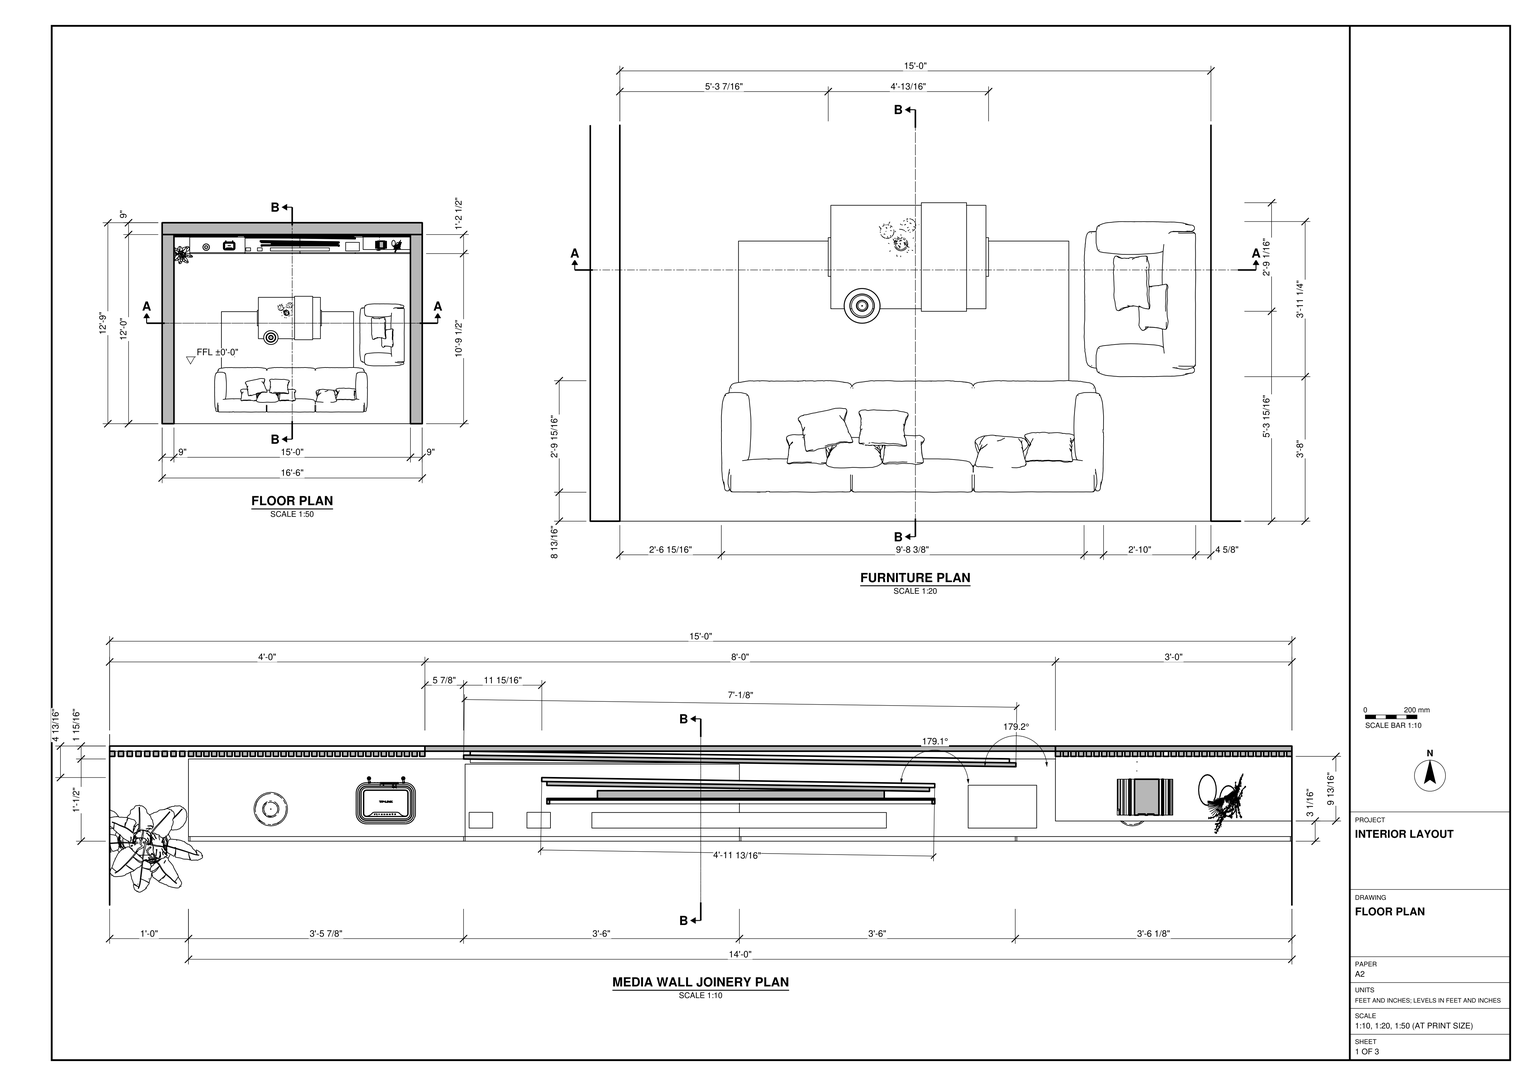
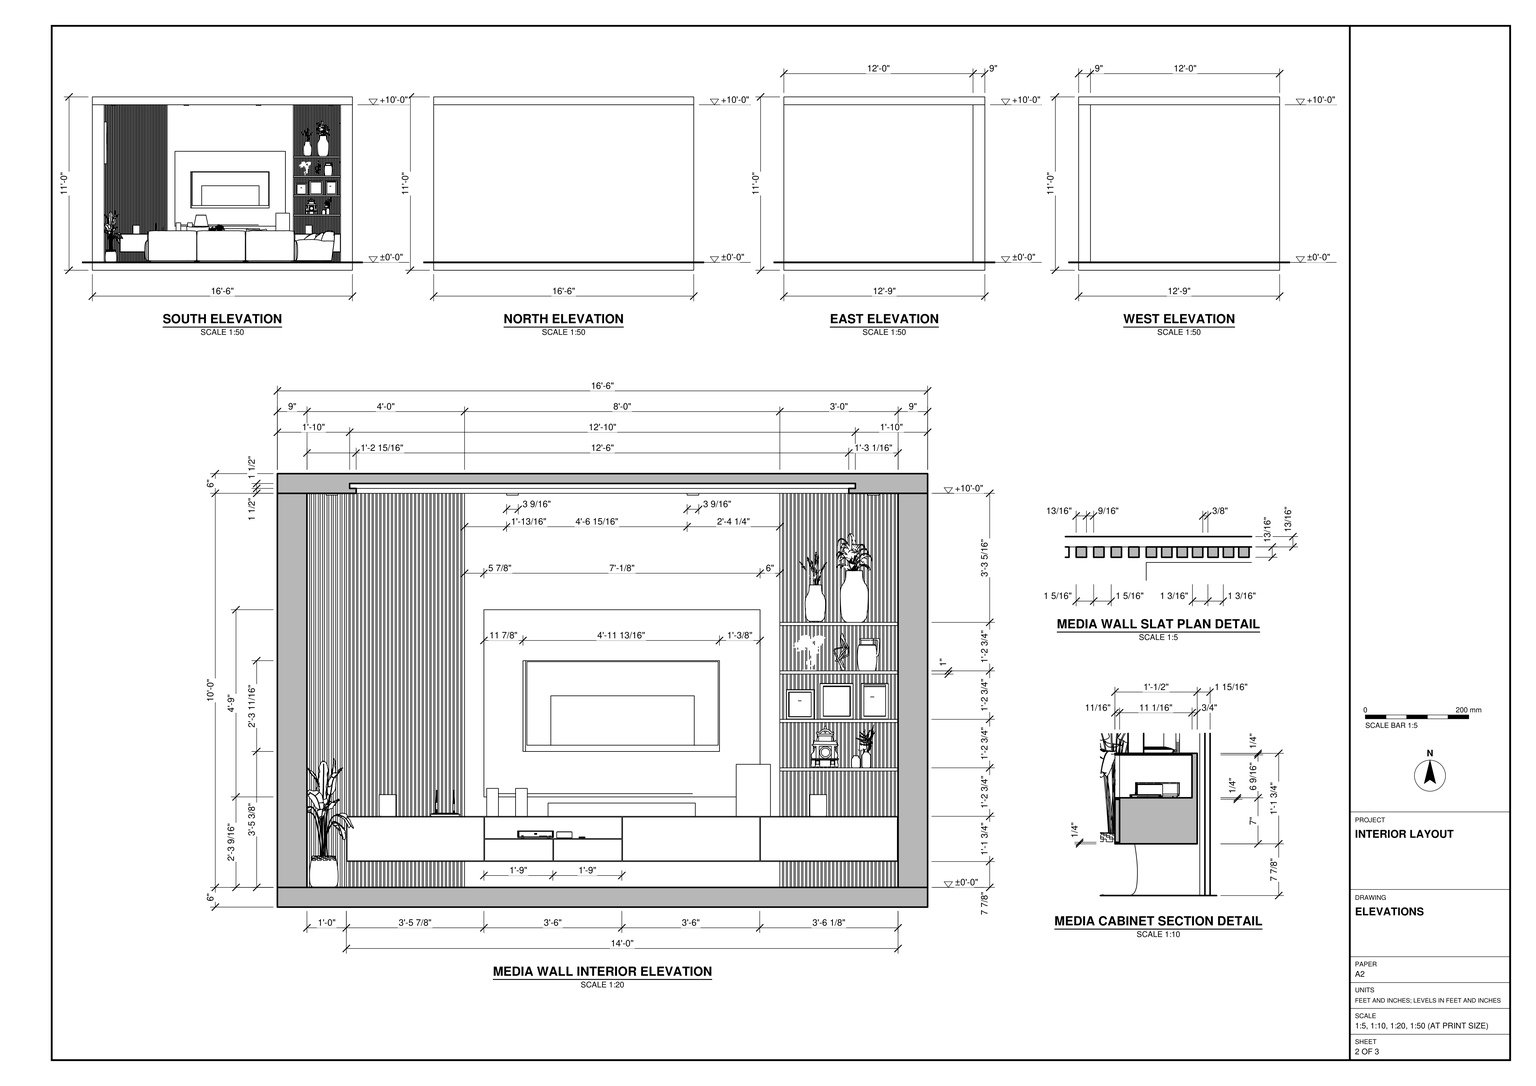
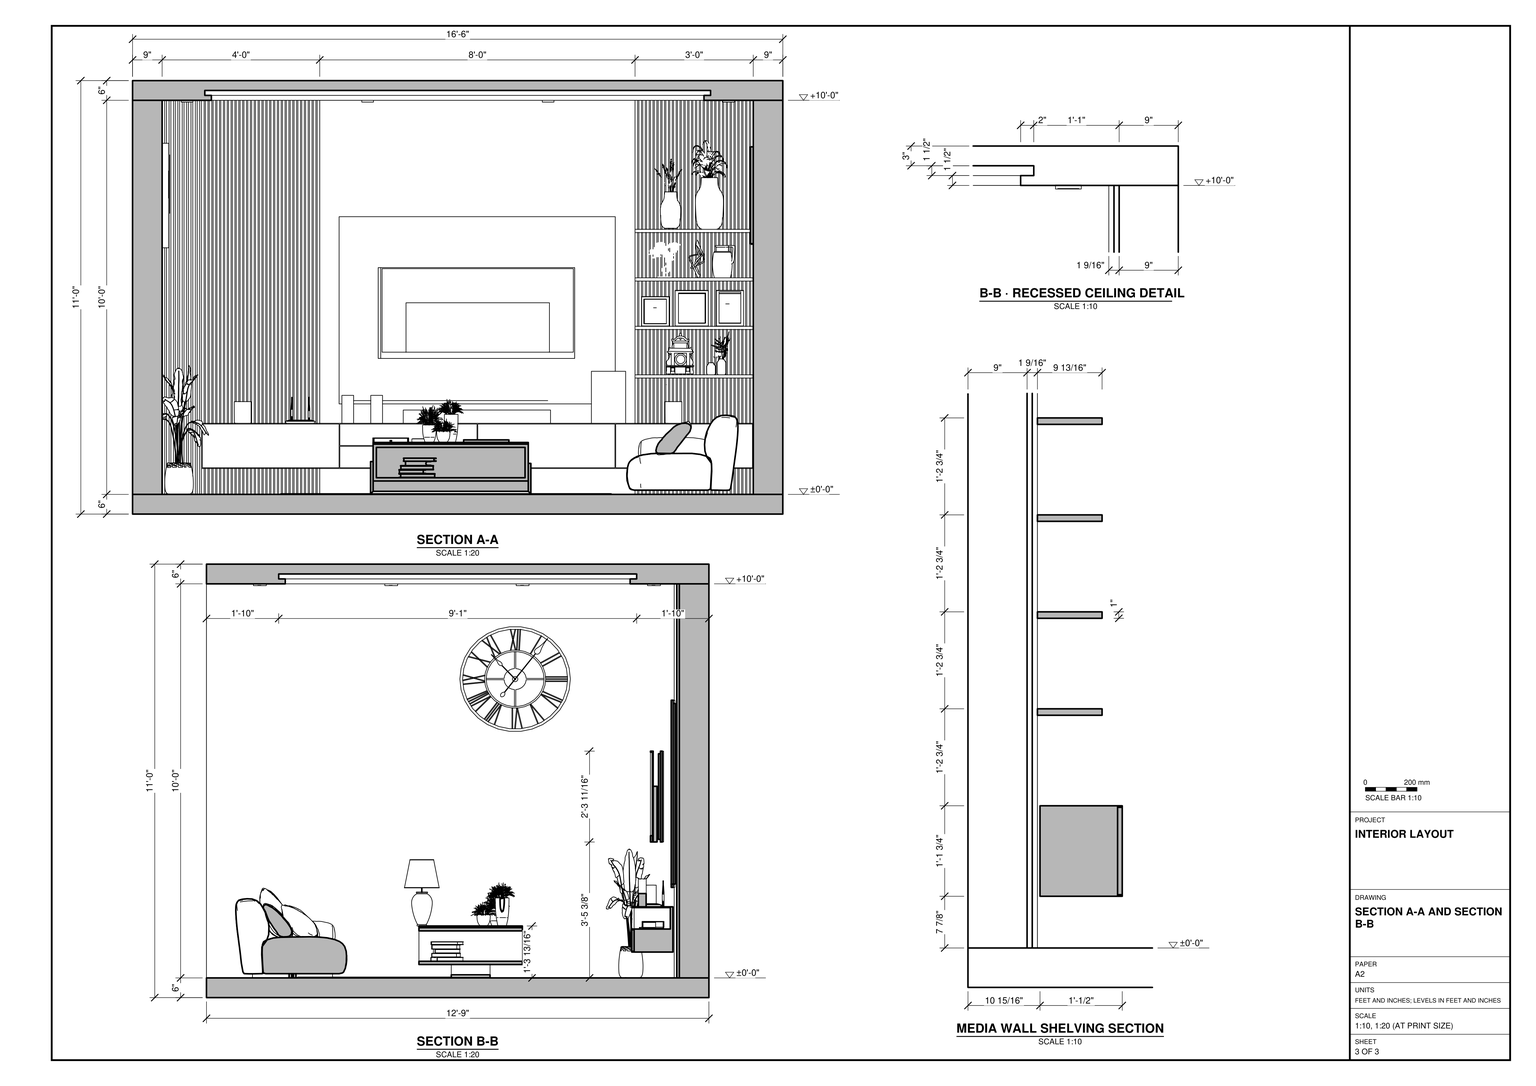
Build the living room in SketchUp using task_files/diagram_01.pdf. Work in feet and inches. The overall shell is 16'-6" wide, 12'-9" deep and 11'-0" high, with the finished floor at ±0'-0". Model the 9" back and side walls, leaving the south side open as drawn. Include the floor slab and ceiling slab, with the main ceiling underside at +10'-0". Use the sections to form the stepped edge of the ceiling recess.

Build the media joinery across the back wall. Place the screen on its backing panel between the two fields of vertical slats. Run the floating cabinet below it, matching the front divisions and open equipment compartment in the interior elevation. Fit the display shelves across the right-hand slatted bay. Use the furniture plan to size and position the sofa facing the screen, the armchair turned towards the coffee table and the low table between the sofa and the media cabinet.

Decor and loose items, including the rug, cushions, plants, clock, lamp and shelf objects, may be any suitable library components placed as shown. Keep the shell elements and each furniture or joinery piece in separate groups or components, and use components for repeated parts. Save one SketchUp model as output_files/furnished_living_room_with_a_built_in_media_wall.skp.

# SketchUp Ruby script. Lengths in inches.
U = 1.inch
M = Sketchup.active_model
def pt(a) = Geom::Point3d.new(a.map { |v| v * U })
def face(e, loops, mat)
  f = e.add_face(loops[0].map { |a| pt(a) })
  loops[1..].each { |l| e.add_face(l.map { |a| pt(a) }).erase! }
  f.material = f.back_material = mat if mat
  f
end
# faces: each face lists its corners as indices into pts; further lists are holes
def faces(e, pts, list, mat = nil) = list.each { |f| face(e, (f[0].is_a?(Array) ? f : [f]).map { |l| l.map { |i| pts[i] } }, mat) }
# xy, xz, yz: faces in a plane at the given z, y or x. An outline is a flat list of corners, or four numbers for a rectangle; further outlines are holes
def ring(l) = l.size == 4 ? [[l[0], l[1]], [l[2], l[1]], [l[2], l[3]], [l[0], l[3]]] : l.each_slice(2).to_a
def flat(e, list, mat, &to3) = list.each { |f| face(e, (f[0].is_a?(Array) ? f : [f]).map { |l| ring(l).map { |u, v| to3.(u, v) } }, mat) }
def xy(e, z, list, mat = nil) = flat(e, list, mat) { |x, y| [x, y, z] }
def xz(e, y, list, mat = nil) = flat(e, list, mat) { |x, z| [x, y, z] }
def yz(e, x, list, mat = nil) = flat(e, list, mat) { |y, z| [x, y, z] }
def lines(e, pts, list) = list.each { |a, b| e.add_line(pt(pts[a]), pt(pts[b])) }
# prism: a flat outline (further loops are holes) pulled along v
def prism(e, loops, v, mat = nil)
  f = face(e, loops, mat); d = Geom::Vector3d.new(v.map { |x| x * U })
  f.pushpull(f.normal.samedirection?(d) ? d.length : -d.length)
end
def box(e, o, s, mat = nil) = prism(e, [[o, [o[0] + s[0], o[1], o[2]], [o[0] + s[0], o[1] + s[1], o[2]], [o[0], o[1] + s[1], o[2]]]], [0, 0, s[2]], mat)
def at(x, y, z, deg = 0) = Geom::Transformation.translation(pt([x, y, z])) * Geom::Transformation.rotation(ORIGIN, Z_AXIS, deg.degrees)
def axes(o, x, y, z) = Geom::Transformation.new([*x, 0, *y, 0, *z, 0, *pt(o).to_a, 1])
def part(name) = M.definitions.add(name)
# library, detail: a bought-in or finely detailed component or shape, given as its bounding box
def library(name, o, s) = part(name).tap { |d| box(d.entities, o, s) }
def detail(e, o, s) = box(e.add_group.entities, o, s)
def put(e, d, t, mat = nil) = e.add_instance(d, t).tap { |i| i.material = mat if mat }
def group(e, t, mat = nil) = e.add_group.tap { |g| g.transformation = t; g.material = mat if mat }.entities
root = M.entities
M.materials.add("1").color = [42, 42, 42]
M.materials.add("2").color = [36, 36, 36]
M.materials.add("20220226_114039").color = [170, 165, 158]
M.materials.add("20220301_203726").color = [120, 123, 130]
M.materials.add("20220304_201918").color = [228, 229, 216]
M.materials.add("3").color = [67, 67, 67]
M.materials.add("Charcoal Blue").color = [36, 31, 24]
M.materials.add("Marble Beige 23-58 150cm").color = [206, 178, 147]
M.materials.add("Marble White SSS 100cm").color = [222, 222, 222]
M.materials.add("PDM_Books_04_Charcoal").color = [35, 35, 35]
M.materials.add("PDM_Books_04_Color_000").color = [255, 255, 255]
M.materials.add("PDM_Books_04_Color_D05").color = [255, 242, 204]
M.materials.add("PDM_Books_04_Material27").color = [78, 78, 71]
M.materials.add("PDM_Books_04_Material30").color = [128, 128, 127]
M.materials.add("PDM_Books_04_Material36").color = [212, 187, 166]
M.materials.add("PDM_Books_04_Material37").color = [155, 160, 155]
M.materials.add("PDM_Books_04_Material8").color = [90, 92, 88]
M.materials.add("Textile_Coffee").color = [176, 143, 74]
M.materials.add("Textile_Ornate_Crimson").color = [133, 75, 58]
M.materials.add("Textile_Pattern_Leopard").color = [156, 141, 132]
M.materials.add("Textile_Salmon").color = [225, 160, 112]
M.materials.add("Tiles Marble Orange 01 160cm").color = [230, 204, 174]
M.materials.add("X15").color = [71, 69, 59]
M.materials.add("[0043_SaddleBrown]").color = [139, 69, 19]
M.materials.add("[0054_LightYellow]").color = [255, 255, 224]
M.materials.add("[0117_GhostWhite]").color = [248, 248, 255]
M.materials.add("[0136_Charcoal]2").color = [35, 35, 35]
M.materials.add("[Blacktop Old 01]").color = [132, 136, 139]
M.materials.add("[Color_E05]").color = [134, 134, 134]
M.materials.add("[Wood Veneer 01]").color = [120, 70, 37]
c1 = part("Area rug")
box(c1.entities,[0,0,0],[137.8,78.74,0.2],"[Color_E05]")
c2 = library("CT-4",[-0.79,-0.79,0],[48.82,34.49,28.93])
c3 = library("Modern-sofa",[28.94,55.09,0],[144.45,82.43,27.34])
c4 = library("Strelitzia Nicolai",[-10.28,-11.9,0],[67.71,67.02,67.96])
c5 = library("skp7CF",[-21.49,-10.21,-1.17],[38.48,21.91,32.59])
c6 = library("modernbiomorphicsculpture",[-2.33,-4.54,0],[48.86,29.63,71.125])
c7 = library("modern sculpture",[-36.1,-27.44,-1.15],[66.07,57.04,107.04])
c8 = library("ABAJUR VIETNAMITA 1",[0,0,0],[17.48,17.48,28.07])
c9 = library("clock",[0.09,-1.71,0],[10.14,8.1,18.46])
c10 = part("Standing picture frame")
yz(c10.entities,0,[[0.272,0,0.522,0.006,0.25,12.003,0,11.997]],"Charcoal Blue")
yz(c10.entities,1,[[0.25,1,0.023,10.997,0.183,11.001,0.375,1.003],[0.375,1.003,0.183,11.001,0.273,11.003,0.499,1.005]],"Charcoal Blue")
yz(c10.entities,9,[[0.25,1,0.375,1.003,0.183,11.001,0.023,10.997],[0.375,1.003,0.499,1.005,0.273,11.003,0.183,11.001]],"Charcoal Blue")
yz(c10.entities,10,[[0.272,0,0,11.997,0.25,12.003,0.522,0.006]],"Charcoal Blue")
p = [[10,0.272,0],[0,0.272,0],[0,0,11.997],[10,0,11.997],[1,0.023,10.997],[1,0.25,1],
  [9,0.25,1],[9,0.023,10.997],[0,0.522,0.006],[10,0.522,0.006],[10,0.25,12.003],[0,0.25,12.003],
  [1,0.499,1.005],[1,0.273,11.003],[9,0.273,11.003],[9,0.499,1.005],[1,0.375,1.002],[9,0.375,1.002],
  [9,0.375,1.003],[9,0.183,11.001],[9,0.173,11.556],[1,0.173,11.556],[1,0.183,11.001],[1,0.375,1.003],
  [1.862,3.823,3.755],[5.256,0.51,7.633],[6.56,0.51,7.633],[3.302,5.095,2.265],[1.862,5.095,2.265]]
faces(c10.entities,p,[[[0,1,2,3],[4,5,6,7]],[[8,9,10,11],[12,13,14,15]],[9,8,1,0],[12,15,18,6,5,23],[14,13,22,4,7,19],[11,10,3,2]],"Charcoal Blue")
faces(c10.entities,p,[[16,17,18,19,20,21,22,23]],"20220304_201918")
faces(c10.entities,p,[[13,12,15,14],[24,25,26,27,28]],"Textile_Coffee")
c11 = part("Standing picture frame \#2")
xy(c11.entities,11,[[1.22,0.02,10.98,0.27]],"Textile_Ornate_Crimson")
xy(c11.entities,12,[[0,0,12.2,0.25]],"Textile_Ornate_Crimson")
yz(c11.entities,0,[[0.27,0,0.52,0.01,0.25,12,0,12]],"Textile_Ornate_Crimson")
yz(c11.entities,1.22,[[0.25,1,0.02,11,0.27,11,0.5,1.01]],"Textile_Ornate_Crimson")
yz(c11.entities,10.98,[[0.25,1,0.5,1.01,0.27,11,0.02,11]],"Textile_Ornate_Crimson")
yz(c11.entities,12.2,[[0.27,0,0,12,0.25,12,0.52,0.01]],"Textile_Ornate_Crimson")
p = [[12.2,0.27,0],[0,0.27,0],[0,0,12],[12.2,0,12],[1.22,0.02,11],[1.22,0.25,1],
  [10.98,0.25,1],[10.98,0.02,11],[0,0.52,0.01],[12.2,0.52,0.01],[12.2,0.25,12],[0,0.25,12],
  [1.22,0.5,1.01],[1.22,0.27,11],[10.98,0.27,11],[10.98,0.5,1.01],[1,0.375,1.01],[10.98,0.375,1.01],
  [10.98,0.1,11],[10.98,0.09,11.15],[1,0.09,11.15],[2.26,3.82,3.75],[5.65,0.51,7.63],[6.95,0.51,7.63],
  [3.7,5.09,2.27],[2.26,5.09,2.27]]
faces(c11.entities,p,[[[0,1,2,3],[4,5,6,7]],[[8,9,10,11],[12,13,14,15]],[9,8,1,0],[12,15,6,5]],"Textile_Ornate_Crimson")
faces(c11.entities,p,[[16,17,18,19,20]],"20220226_114039")
faces(c11.entities,p,[[13,12,15,14],[21,22,23,24,25]],"Textile_Pattern_Leopard")
c12 = part("Standing picture frame \#1")
xy(c12.entities,11,[[1.22,0.02,10.98,0.08],[1.22,0.08,10.98,0.27]],"Textile_Salmon")
xy(c12.entities,12,[[0,0,12.2,0.25]],"Textile_Salmon")
yz(c12.entities,0,[[0.27,0,0.52,0.01,0.25,12,0,12]],"Textile_Salmon")
yz(c12.entities,1.22,[[0.25,1,0.02,11,0.27,11,0.5,1.01]],"Textile_Salmon")
yz(c12.entities,10.98,[[0.25,1,0.5,1.01,0.27,11,0.02,11]],"Textile_Salmon")
yz(c12.entities,12.2,[[0.27,0,0,12,0.25,12,0.52,0.01]],"Textile_Salmon")
p = [[12.2,0.27,0],[0,0.27,0],[0,0,12],[12.2,0,12],[1.22,0.02,11],[1.22,0.25,1],
  [10.98,0.25,1],[10.98,0.02,11],[0,0.52,0.01],[12.2,0.52,0.01],[12.2,0.25,12],[0,0.25,12],
  [1.22,0.5,1.01],[1.22,0.27,11],[10.98,0.27,11],[10.98,0.5,1.01],[1.22,0.36,1.01],[11.29,0.36,1.01],
  [11.29,0.08,11],[10.98,0.08,11],[1.22,0.08,11],[2.26,3.82,3.75],[5.65,0.51,7.63],[6.95,0.51,7.63],
  [3.7,5.09,2.27],[2.26,5.09,2.27]]
faces(c12.entities,p,[[[0,1,2,3],[4,5,6,7]],[[8,9,10,11],[12,13,14,15]],[9,8,1,0],[12,15,6,5],[13,12,15,14],[21,22,23,24,25]],"Textile_Salmon")
faces(c12.entities,p,[[16,17,18,19,20]],"20220301_203726")
c13 = part("cadres")
put(c13.entities,c10,axes([3.21,-0.47,0.23],[1,0,0],[0,0.89337,-0.44932],[0,0.44932,0.89337]))
put(c13.entities,c11,axes([16.15,-0.47,0.23],[1,0,0],[0,0.89337,-0.44932],[0,0.44932,0.89337]))
put(c13.entities,c12,axes([30.57,-0.39,0.19],[0.8272,0,0],[0,0.739,-0.37168],[0,0.37168,0.739]))
c14 = library("Candle 293 010 003",[-2.56,-2.56,-0.02],[5.11,5.12,6.62])
c15 = library("Jug",[-0.64,0.09,0],[6.72,6.82,9.84])
c16 = part("Books_04_component_01")
xy(c16.entities,0,[[0.04,0,0,0.04,0,7.875,0.12,7.875,0.12,0.24,1.25,0.24,1.25,7.875,1.36,7.875,1.36,0.04,1.3125,0]],"PDM_Books_04_Color_000")
xy(c16.entities,0.11,[[0.12,0.24,0.12,7.76,0.21,7.74,0.3,7.73,0.4,7.73,0.49,7.72,0.87,7.72,0.96,7.73,1.06,7.73,1.15,7.74,1.25,7.76,1.25,0.24]],"PDM_Books_04_Color_D05")
xy(c16.entities,8.99,[[0.12,0.12,1.25,0.12,1.25,7.76,1.15,7.74,1.06,7.73,0.96,7.73,0.87,7.72,0.49,7.72,0.4,7.73,0.3,7.73,0.21,7.74,0.12,7.76]],"PDM_Books_04_Color_D05")
xy(c16.entities,9.1,[[0.04,0,1.3125,0,1.36,0.04,1.36,7.875,1.25,7.875,1.25,0.12,0.12,0.12,0.12,7.875,0,7.875,0,0.04]],"PDM_Books_04_Color_000")
xz(c16.entities,0,[[0.04,0,1.3125,9.1]],"PDM_Books_04_Material36")
xz(c16.entities,0.12,[[0.12,8.99,1.25,9.1]],"PDM_Books_04_Color_000")
xz(c16.entities,0.24,[[0.12,0,1.25,0.11]],"PDM_Books_04_Color_000")
xz(c16.entities,7.72,[[0.49,0.11,0.59,8.99],[0.59,0.11,0.68,8.99],[0.68,0.11,0.78,8.99],[0.78,0.11,0.87,8.99]],"PDM_Books_04_Color_D05")
xz(c16.entities,7.73,[[0.3,0.11,0.4,8.99],[0.96,0.11,1.06,8.99]],"PDM_Books_04_Color_D05")
xz(c16.entities,7.875,[[0,0,0.12,9.1],[1.25,0,1.36,9.1]],"PDM_Books_04_Color_000")
yz(c16.entities,0,[[0.04,0,7.875,9.1]],"PDM_Books_04_Material36")
yz(c16.entities,0.12,[[0.24,0,7.875,0,7.875,9.1,0.12,9.1,0.12,8.99,7.76,8.99,7.76,0.11,0.24,0.11]],"PDM_Books_04_Color_000")
yz(c16.entities,1.25,[[0.24,0,0.24,0.11,7.76,0.11,7.76,8.99,0.12,8.99,0.12,9.1,7.875,9.1,7.875,0]],"PDM_Books_04_Color_000")
yz(c16.entities,1.36,[[0.04,0,7.875,9.1]],"PDM_Books_04_Material36")
p = [[0.04,0,0],[0.04,0,9.1],[0,0.04,9.1],[0,0.04,0],[1.3125,0,9.1],[1.3125,0,0],
  [1.36,0.04,0],[1.36,0.04,9.1],[0.21,7.74,0.11],[0.12,7.76,0.11],[0.12,7.76,8.99],[0.21,7.74,8.99],
  [0.3,7.73,0.11],[0.3,7.73,8.99],[0.49,7.72,0.11],[0.4,7.73,0.11],[0.4,7.73,8.99],[0.49,7.72,8.99],
  [0.96,7.73,0.11],[0.87,7.72,0.11],[0.87,7.72,8.99],[0.96,7.73,8.99],[1.15,7.74,0.11],[1.06,7.73,0.11],
  [1.06,7.73,8.99],[1.15,7.74,8.99],[1.25,7.76,0.11],[1.25,7.76,8.99]]
faces(c16.entities,p,[[0,1,2,3],[4,5,6,7]],"PDM_Books_04_Material36")
faces(c16.entities,p,[[8,9,10,11],[12,8,11,13],[14,15,16,17],[18,19,20,21],[22,23,24,25],[26,22,25,27]],"PDM_Books_04_Color_D05")
c17 = part("Books_04_component_05")
xy(c17.entities,0,[[0.04,0,0,0.04,0,8.31,0.12,8.31,0.12,0.24,0.83,0.18,0.83,8.31,0.94,8.31,0.94,0.04,0.9,0]],"PDM_Books_04_Color_000")
xy(c17.entities,0.11,[[0.83,0.18,0.12,0.24,0.12,8.1875,0.17,8.18,0.23,8.18,0.29,8.17,0.35,8.17,0.41,8.16,0.53,8.16,0.59,8.17,0.65,8.17,0.71,8.18,0.77,8.18,0.83,8.1875]],"PDM_Books_04_Color_D05")
xy(c17.entities,9.65,[[0.12,0.24,0.83,0.24,0.83,8.1875,0.77,8.18,0.71,8.18,0.65,8.17,0.59,8.17,0.53,8.16,0.41,8.16,0.35,8.17,0.29,8.17,0.23,8.18,0.17,8.18,0.12,8.1875]],"PDM_Books_04_Color_D05")
xy(c17.entities,9.76,[[0.04,0,0.9,0,0.94,0.04,0.94,8.31,0.83,8.31,0.83,0.24,0.12,0.24,0.12,8.31,0,8.31,0,0.04]],"PDM_Books_04_Color_000")
xz(c17.entities,0,[[0.04,0,0.9,9.76]],"PDM_Books_04_Material37")
xz(c17.entities,0.24,[[0.12,9.65,0.83,9.76]],"PDM_Books_04_Color_000")
xz(c17.entities,8.16,[[0.41,0.11,0.47,9.65],[0.47,0.11,0.53,9.65]],"PDM_Books_04_Color_D05")
xz(c17.entities,8.17,[[0.29,0.11,0.35,9.65],[0.59,0.11,0.65,9.65]],"PDM_Books_04_Color_D05")
xz(c17.entities,8.18,[[0.17,0.11,0.23,9.65],[0.71,0.11,0.77,9.65]],"PDM_Books_04_Color_D05")
xz(c17.entities,8.31,[[0,0,0.12,9.76],[0.83,0,0.94,9.76]],"PDM_Books_04_Color_000")
yz(c17.entities,0,[[0.04,0,8.31,9.76]],"PDM_Books_04_Material37")
yz(c17.entities,0.12,[[0.24,0,8.31,0,8.31,9.76,0.24,9.76,0.24,9.65,8.1875,9.65,8.1875,0.11,0.24,0.11]],"PDM_Books_04_Color_000")
yz(c17.entities,0.83,[[0.18,0,0.18,0.11,8.1875,0.11,8.1875,9.65,0.24,9.65,0.24,9.76,8.31,9.76,8.31,0]],"PDM_Books_04_Color_000")
yz(c17.entities,0.94,[[0.04,0,8.31,9.76]],"PDM_Books_04_Material37")
p = [[0,0.04,9.76],[0,0.04,0],[0.04,0,0],[0.04,0,9.76],[0.94,0.04,0],[0.94,0.04,9.76],
  [0.9,0,9.76],[0.9,0,0],[0.83,0.18,0.11],[0.83,0.18,0],[0.12,0.24,0],[0.12,0.24,0.11],
  [0.12,8.1875,0.11],[0.12,8.1875,9.65],[0.17,8.18,9.65],[0.17,8.18,0.11],[0.29,8.17,0.11],[0.23,8.18,0.11],
  [0.23,8.18,9.65],[0.29,8.17,9.65],[0.41,8.16,0.11],[0.35,8.17,0.11],[0.35,8.17,9.65],[0.41,8.16,9.65],
  [0.59,8.17,0.11],[0.53,8.16,0.11],[0.53,8.16,9.65],[0.59,8.17,9.65],[0.71,8.18,0.11],[0.65,8.17,0.11],
  [0.65,8.17,9.65],[0.71,8.18,9.65],[0.83,8.1875,0.11],[0.77,8.18,0.11],[0.77,8.18,9.65],[0.83,8.1875,9.65]]
faces(c17.entities,p,[[0,1,2,3],[4,5,6,7]],"PDM_Books_04_Material37")
faces(c17.entities,p,[[8,9,10,11]],"PDM_Books_04_Color_000")
faces(c17.entities,p,[[12,13,14,15],[16,17,18,19],[20,21,22,23],[24,25,26,27],[28,29,30,31],[32,33,34,35]],"PDM_Books_04_Color_D05")
c18 = part("Books_04_component_02")
xy(c18.entities,0,[[0.04,0,0,0.04,0,7.67,0.12,7.67,0.12,0.12,1.11,0.12,1.11,7.67,1.22,7.67,1.22,0.04,1.18,0]],"PDM_Books_04_Color_000")
xy(c18.entities,0.08,[[0.12,0.12,1.11,7.59]],"PDM_Books_04_Color_D05")
xy(c18.entities,10.875,[[0.12,0.12,1.11,7.59]],"PDM_Books_04_Color_D05")
xy(c18.entities,10.99,[[0.04,0,1.18,0,1.22,0.04,1.22,7.67,1.11,7.67,1.11,0.12,0.12,0.12,0.12,7.67,0,7.67,0,0.04]],"PDM_Books_04_Color_000")
xz(c18.entities,0,[[0.04,0,1.18,10.99]],"PDM_Books_04_Material8")
xz(c18.entities,0.12,[[0.12,0,1.11,0.08],[0.12,0.08,1.11,10.875]])
xz(c18.entities,0.12,[[0.12,10.875,1.11,10.99]],"PDM_Books_04_Color_000")
xz(c18.entities,7.59,[[0.12,0.08,1.11,10.875]],"PDM_Books_04_Color_D05")
xz(c18.entities,7.67,[[1.11,0,1.22,10.99]],"PDM_Books_04_Color_000")
xz(c18.entities,7.67,[[0,0,0.12,10.99]],"PDM_Books_04_Material8")
yz(c18.entities,0,[[0.04,0,7.67,10.99]],"PDM_Books_04_Material8")
yz(c18.entities,0.12,[[0.12,0,7.67,0,7.67,10.99,0.12,10.99,0.12,10.875,7.59,10.875,7.59,0.08,0.12,0.08]])
yz(c18.entities,0.12,[[0.12,0.08,7.59,10.875]],"PDM_Books_04_Material8")
yz(c18.entities,1.11,[[0.12,0,0.12,0.08,7.59,0.08,7.59,10.875,0.12,10.875,0.12,10.99,7.67,10.99,7.67,0],[0.12,0.08,7.59,10.875]])
yz(c18.entities,1.22,[[0.04,0,7.67,10.99]],"PDM_Books_04_Material8")
p = [[0,0.04,10.99],[0,0.04,0],[0.04,0,0],[0.04,0,10.99],[1.22,0.04,0],[1.22,0.04,10.99],
  [1.18,0,10.99],[1.18,0,0]]
faces(c18.entities,p,[[0,1,2,3],[4,5,6,7]],"PDM_Books_04_Material8")
c19 = part("Books_04_component_03")
xy(c19.entities,0,[[0.04,0,0,0.04,0,7.67,0.12,7.67,0.12,0.12,1.11,0.12,1.11,7.67,1.22,7.67,1.22,0.04,1.18,0]],"PDM_Books_04_Color_000")
xy(c19.entities,0.08,[[0.12,0.12,1.11,7.59]],"PDM_Books_04_Color_D05")
xy(c19.entities,9.89,[[0.12,0.12,1.11,7.59]],"PDM_Books_04_Color_D05")
xy(c19.entities,10,[[0.04,0,1.18,0,1.22,0.04,1.22,7.67,1.11,7.67,1.11,0.12,0.12,0.12,0.12,7.67,0,7.67,0,0.04]],"PDM_Books_04_Color_000")
xz(c19.entities,0,[[0.04,7.99,1.18,10]],"PDM_Books_04_Color_000")
xz(c19.entities,0,[[0.04,0,1.18,7.99]],"PDM_Books_04_Material30")
xz(c19.entities,0.12,[[0.12,0,1.11,0.08],[0.12,0.08,1.11,9.89]])
xz(c19.entities,0.12,[[0.12,9.89,1.11,10]],"PDM_Books_04_Color_000")
xz(c19.entities,7.59,[[0.12,0.08,1.11,9.89]],"PDM_Books_04_Color_D05")
xz(c19.entities,7.67,[[1.11,0,1.22,10]],"PDM_Books_04_Color_000")
xz(c19.entities,7.67,[[0,0,0.12,10]],"PDM_Books_04_Material8")
yz(c19.entities,0,[[0.04,0,7.67,10]],"PDM_Books_04_Material30")
yz(c19.entities,0.12,[[0.12,0,7.67,0,7.67,10,0.12,10,0.12,9.89,7.59,9.89,7.59,0.08,0.12,0.08]])
yz(c19.entities,0.12,[[0.12,0.08,7.59,9.89]],"PDM_Books_04_Material8")
yz(c19.entities,1.11,[[0.12,0,0.12,0.08,7.59,0.08,7.59,9.89,0.12,9.89,0.12,10,7.67,10,7.67,0],[0.12,0.08,7.59,9.89]])
yz(c19.entities,1.22,[[0.04,0,7.67,10]],"PDM_Books_04_Material30")
p = [[0.04,0,0],[0.04,0,7.99],[0,0.04,7.99],[0,0.04,0],[1.18,0,7.99],[1.18,0,0],
  [1.22,0.04,0],[1.22,0.04,7.99],[0.04,0,10],[0,0.04,10],[1.18,0,10],[1.22,0.04,10]]
faces(c19.entities,p,[[0,1,2,3],[4,5,6,7]],"PDM_Books_04_Material30")
faces(c19.entities,p,[[1,8,9,2],[10,4,7,11]],"PDM_Books_04_Color_000")
c20 = part("Books_04_component_04")
xy(c20.entities,0,[[0.04,0,0,0.04,0,8.1,0.12,8.1,0.12,0.12,1.11,0.12,1.11,8.1,1.22,8.1,1.22,0.04,1.18,0]],"PDM_Books_04_Color_000")
xy(c20.entities,0.08,[[0.12,0.12,1.11,8.02]],"PDM_Books_04_Color_D05")
xy(c20.entities,11.98,[[0.12,0.12,1.11,8.02]],"PDM_Books_04_Color_D05")
xy(c20.entities,12.09,[[0.04,0,1.18,0,1.22,0.04,1.22,8.1,1.11,8.1,1.11,0.12,0.12,0.12,0.12,8.1,0,8.1,0,0.04]],"PDM_Books_04_Color_000")
xz(c20.entities,0,[[0.04,7.96,1.18,12.09]],"PDM_Books_04_Charcoal")
xz(c20.entities,0,[[0.04,0,1.18,7.96]],"PDM_Books_04_Material27")
xz(c20.entities,0.12,[[0.12,0,1.11,0.08],[0.12,0.08,1.11,11.98]])
xz(c20.entities,0.12,[[0.12,11.98,1.11,12.09]],"PDM_Books_04_Color_000")
xz(c20.entities,8.02,[[0.12,0.08,1.11,11.98]],"PDM_Books_04_Color_D05")
xz(c20.entities,8.1,[[1.11,0,1.22,12.09]],"PDM_Books_04_Color_000")
xz(c20.entities,8.1,[[0,0,0.12,12.09]],"PDM_Books_04_Material8")
yz(c20.entities,0,[[0.04,0,8.1,12.09]],"PDM_Books_04_Material27")
yz(c20.entities,0.12,[[0.12,0,8.1,0,8.1,12.09,0.12,12.09,0.12,11.98,8.02,11.98,8.02,0.08,0.12,0.08]])
yz(c20.entities,0.12,[[0.12,0.08,8.02,11.98]],"PDM_Books_04_Material8")
yz(c20.entities,1.11,[[0.12,0,0.12,0.08,8.02,0.08,8.02,11.98,0.12,11.98,0.12,12.09,8.1,12.09,8.1,0],[0.12,0.08,8.02,11.98]])
yz(c20.entities,1.22,[[0.04,0,8.1,12.09]],"PDM_Books_04_Material27")
p = [[0,0.04,7.96],[0,0.04,0],[0.04,0,0],[0.04,0,7.96],[1.18,0,7.96],[1.18,0,0],
  [1.22,0.04,0],[1.22,0.04,7.96],[0,0.04,12.09],[0.04,0,12.09],[1.18,0,12.09],[1.22,0.04,12.09]]
faces(c20.entities,p,[[0,1,2,3],[4,5,6,7]],"PDM_Books_04_Material27")
faces(c20.entities,p,[[8,0,3,9],[10,4,7,11]],"PDM_Books_04_Charcoal")
c21 = part("Book")
put(c21.entities,c16,axes([4.875,-4.73,3.67],[0,0,1],[0.10106,0.99488,0],[-0.99488,0.10106,0]))
put(c21.entities,c17,axes([4.5,-4.91,5.03],[0,0,1],[0.17365,0.98481,0],[-0.98481,0.17365,0]))
put(c21.entities,c18,axes([4.85,-4.7,1.22],[0,0,1],[0.108,0.99415,0],[-0.99415,0.108,0]))
put(c21.entities,c19,axes([5.47,-3.69,2.45],[0,0,1],[-0.04711,0.99889,0],[-0.99889,-0.04711,0]))
put(c21.entities,c20,axes([6.6,-3.07,0],[0,0,1],[-0.15643,0.98769,0],[-0.98769,-0.15643,0]))
c22 = library("SET TOP BOX",[-9.27,3.26,0],[16.98,7.55,1.57])
c23 = library("ROUTER WIFI",[-18.49,16.54,21.65],[9.06,7.22,7.96])
c24 = library("Decor Vase Bowl (19)",[0,-5.46,0],[24.42,18.18,42.16])
c25 = part("Sound bar\#1")
xy(c25.entities,0,[[0,0,35.43,3.54]])
xy(c25.entities,2.52,[[0,0,35.43,3.54]])
xz(c25.entities,0,[[0,0,35.43,2.52]],"3")
xz(c25.entities,3.54,[[0,0,35.43,2.52]])
yz(c25.entities,0,[[0,0,3.54,2.52]])
yz(c25.entities,35.43,[[0,0,3.54,2.52]])
c26 = part("Subwoofer speaker")
xy(c26.entities,0,[[0,0,8.15,12.99]])
xy(c26.entities,15.83,[[0,0,8.15,12.99]],"[0136_Charcoal]2")
xz(c26.entities,0,[[0,0,8.15,15.83]],"2")
xz(c26.entities,12.99,[[0,0,8.15,15.83]],"[0136_Charcoal]2")
yz(c26.entities,0,[[0,0,12.99,15.83]],"[0136_Charcoal]2")
yz(c26.entities,8.15,[[0,0,12.99,15.83]],"[0136_Charcoal]2")
c27 = part("Satellite speaker")
xy(c27.entities,0,[[0,0,3.58,3.58]])
xy(c27.entities,8.5,[[0,0,3.58,3.58]])
xz(c27.entities,0,[[0,0,3.58,8.5]],"1")
xz(c27.entities,3.58,[[0,0,3.58,8.5]])
yz(c27.entities,0,[[0,0,3.58,8.5]])
yz(c27.entities,3.58,[[0,0,3.58,8.5]])
c28 = part("Sound bar3")
put(c28.entities,c25,axes([17.92,0,0],[1.2656,0,0],[0,1,0],[0,0,1.6]),"[0136_Charcoal]2")
put(c28.entities,c26,axes([75.21,0,0],[1.28,0,0],[0,0.75,0],[0,0,1]))
put(c28.entities,c27,at(-0.77,0,0),"[0136_Charcoal]2")
put(c28.entities,c27,at(8.03,0,0),"[0136_Charcoal]2")
c29 = library("METAL FRAME WALL CLOCK",[38.26,45.66,75.01],[15.95,0.53,15.86])
c30 = library("Ceiling Light Fixture",[-0.01,-0.05,0.16],[4.49,4.78,0.61])
c31 = part("X1")
xz(c31.entities,3782.5625,[[3162.97,-138.39,6295.89,0.79]],"X15")
xz(c31.entities,3818.59,[[6779.68,-138.39,9858.78,0.79]],"X15")
g1 = group(c31.entities,at(3162.97,3782.5625,-138.39))
xy(g1,139.17,[[0,0,3132.91,4125.39],[3616.71,36.03,6695.81,4113.24],[7124.85,56.49,10192.6,4117.87]],"X15")
xz(g1,56.49,[[7124.85,0,10192.6,139.17]],"X15")
xz(g1,4113.24,[[3616.71,0,6695.81,139.17]],"X15")
xz(g1,4117.87,[[7124.85,0,10192.6,139.17]],"X15")
xz(g1,4125.39,[[0,0,3132.91,139.17]],"X15")
yz(g1,0,[[0,0,4125.39,139.17]],"X15")
yz(g1,3132.91,[[0,0,4125.39,139.17]],"X15")
yz(g1,3616.71,[[36.03,0,4113.24,139.17]],"X15")
yz(g1,6695.81,[[36.03,0,4113.24,139.17]],"X15")
yz(g1,7124.85,[[56.49,0,4117.87,139.17]],"X15")
yz(g1,10192.6,[[56.49,0,4117.87,139.17]],"X15")
c32 = part("Group\#5")
box(c32.entities,[0,-0.79,0],[0.79,0.79,120])
c33 = part("52a36b60-1cdb-40d2-a4ac-907526ab5b00:a80701cd-a097-4bc1-819a")
xy(c33.entities,2.56,[[-14.15,-1,-14.15,-0.41,14.15,-0.41],[-14.15,-1,14.15,-0.41,14.15,-1],[-14.15,-0.41,-14.15,-0.18,14.15,-0.18],[-14.15,-0.41,14.15,-0.18,14.15,-0.41],[-10.47,-0.18,-10.47,1,10.47,1],
  [-10.47,-0.18,10.47,1,10.47,-0.18]])
xy(c33.entities,3.74,[[-13.96,-1,13.96,-1,-13.96,-0.41],[13.96,-1,13.96,-0.41,-13.96,-0.41]])
xy(c33.entities,13.03,[[-10.47,-0.18,10.47,-0.18,-10.47,1],[10.47,-0.18,10.47,1,-10.47,1]])
xy(c33.entities,19.45,[[-13.96,-1,-13.96,-0.41,13.96,-0.41],[-13.96,-1,13.96,-0.41,13.96,-1]])
xy(c33.entities,19.65,[[-14.15,-1,14.15,-1,-14.15,-0.41],[14.15,-1,14.15,-0.41,-14.15,-0.41],[-14.15,-0.41,14.15,-0.41,-14.15,-0.18],[14.15,-0.41,14.15,-0.18,-14.15,-0.18]])
xz(c33.entities,-1,[[-14.15,2.56,-13.96,3.74,-14.15,19.65],[-14.15,2.56,14.15,2.56,-13.96,3.74],[14.15,2.56,13.96,3.74,-13.96,3.74],[14.15,2.56,14.15,19.65,13.96,3.74],[-13.96,3.74,-13.96,19.45,-14.15,19.65],
  [13.96,3.74,14.15,19.65,13.96,19.45],[-13.96,19.45,13.96,19.45,-14.15,19.65],[13.96,19.45,14.15,19.65,-14.15,19.65]])
xz(c33.entities,-0.41,[[-14.15,2.56,-13.96,3.74,14.15,2.56],[-14.15,2.56,-14.15,19.65,-13.96,3.74],[-14.15,2.56,14.15,2.56,-14.15,19.65],[14.15,2.56,14.15,19.65,-14.15,19.65],[14.15,2.56,-13.96,3.74,13.96,3.74],
  [14.15,2.56,13.96,3.74,14.15,19.65],[-13.96,3.74,-14.15,19.65,-13.96,19.45],[13.96,3.74,13.96,19.45,14.15,19.65],[-13.96,19.45,-14.15,19.65,13.96,19.45],[13.96,19.45,-14.15,19.65,14.15,19.65]])
xz(c33.entities,-0.18,[[-14.15,2.56,-14.15,19.65,14.15,2.56],[14.15,2.56,-14.15,19.65,14.15,19.65],[-10.47,2.56,10.47,2.56,-10.47,13.03],[10.47,2.56,10.47,13.03,-10.47,13.03]])
xz(c33.entities,1,[[-10.47,2.56,-10.47,13.03,10.47,13.03],[-10.47,2.56,10.47,13.03,10.47,2.56]])
yz(c33.entities,-14.15,[[-0.41,2.56,-1,19.65,-0.41,19.65],[-1,2.56,-1,19.65,-0.41,2.56],[-0.18,2.56,-0.41,19.65,-0.18,19.65],[-0.41,2.56,-0.41,19.65,-0.18,2.56]])
yz(c33.entities,-13.96,[[-1,3.74,-0.41,19.45,-1,19.45],[-1,3.74,-0.41,3.74,-0.41,19.45]])
yz(c33.entities,-10.47,[[-0.18,2.56,-0.18,13.03,1,2.56],[1,2.56,-0.18,13.03,1,13.03]])
yz(c33.entities,10.47,[[-0.18,2.56,1,13.03,-0.18,13.03],[-0.18,2.56,1,2.56,1,13.03]])
yz(c33.entities,13.96,[[-0.41,3.74,-1,19.45,-0.41,19.45],[-1,3.74,-1,19.45,-0.41,3.74]])
yz(c33.entities,14.15,[[-1,2.56,-0.41,19.65,-1,19.65],[-1,2.56,-0.41,2.56,-0.41,19.65],[-0.41,2.56,-0.18,19.65,-0.41,19.65],[-0.41,2.56,-0.18,2.56,-0.18,19.65]])
put(root,c1,axes([45.14,27.82,0],[0.73,0,0],[0,0.73,0],[0,0,0.73]))
put(root,c2,at(73.25,64.7,0.14))
put(root,c3,at(213.3,146.34,0,180))
put(root,c4,axes([3.04,125.37,0],[0.38034,-0.13543,0],[0.10841,0.30446,0],[0,0,0.58011]))
put(root,c5,axes([171.08,135.82,81.6875],[0.58721,0,0],[0,0.69,0],[0,0,0.83204]))
put(root,c6,axes([156.79,135.23,65.94],[0.23218,0,0],[0,0.23,0],[0,0,0.15568]))
put(root,c7,axes([171.98,137.27,66.07],[0.07286,0,0],[0,0.0837,0],[0,0,0.10731]))
put(root,c8,axes([77.25,60.24,15.8125],[0.63126,0,0],[0,0.61,0],[0,0,0.72021]))
put(root,c9,axes([162.28,135.1875,33.42],[0.84,0,0],[0,1,0],[0,0,0.85]))
put(root,c13,axes([188.69,134.1875,51.18],[-0.82801,0,0],[0,1,0],[0,0,1]))
put(root,c14,at(164.7,134.4,21.68))
put(root,c14,at(33.53,134.4,21.68))
put(root,c15,at(176.5,139.7,65.94,-90))
put(root,c21,at(86.47,73.26,5.06))
put(root,c22,axes([84.35,128.51,14.88],[1.2099,0,0],[0,1,0],[0,0,1.48]))
put(root,c23,at(37.09,155.89,0,180))
put(root,c24,axes([174.77,132.1875,36.43],[0.35,0,0],[0,0.60706,0],[0,0,0.3103]))
put(root,c28,axes([64.51,131.51,21.65],[1,0,0],[0,0.67,0],[0,0,1]))
put(root,c29,axes([207.61,-3.58,-75.41],[0,2.11,0],[-4.3,0,0],[0,0,2.0064]))
put(root,c30,axes([14.38,13.92,120.23],[1,0,0],[0,1,0],[0,0,-1]))
put(root,c30,axes([69.34,13.92,120.23],[1,0,0],[0,1,0],[0,0,-1]))
put(root,c30,axes([124.3,13.92,120.23],[1,0,0],[0,1,0],[0,0,-1]))
put(root,c30,axes([179.26,13.92,120.23],[1,0,0],[0,1,0],[0,0,-1]))
put(root,c30,axes([14.38,53.92,120.23],[1,0,0],[0,1,0],[0,0,-1]))
put(root,c30,axes([179.26,53.92,120.23],[1,0,0],[0,1,0],[0,0,-1]))
put(root,c30,axes([14.38,93.92,120.23],[1,0,0],[0,1,0],[0,0,-1]))
put(root,c30,axes([179.26,93.92,120.23],[1,0,0],[0,1,0],[0,0,-1]))
put(root,c30,axes([14.38,133.92,120.23],[1,0,0],[0,1,0],[0,0,-1]))
put(root,c30,axes([69.34,133.92,120.23],[1,0,0],[0,1,0],[0,0,-1]))
put(root,c30,axes([179.26,133.92,120.23],[1,0,0],[0,1,0],[0,0,-1]))
put(root,c30,axes([124.3,133.92,120.23],[1,0,0],[0,1,0],[0,0,-1]))
put(root,c31,axes([188.16,120.1,48.71],[0,-0.00599,0],[0,0,0.00723],[-0.00609,0,0]))
g2 = group(root,at(21,142.03,7.875),"[Wood Veneer 01]")
xy(g2,0,[[0,-12.52,168,-11.8125],[0,-11.8125,168,-0.96]])
xy(g2,0.24,[[0.24,-12.52,41.88,-11.8125],[42.12,-12.52,62.88,-11.8125],[63.12,-12.52,83.88,-11.8125],[84.12,-12.52,125.88,-11.8125],[126.12,-12.52,167.76,-11.8125]])
xy(g2,6.77,[[42.12,-12.52,62.88,-11.8125],[63.12,-12.52,83.88,-11.8125]])
xy(g2,7.01,[[42.12,-12.52,83.88,-11.8125],[42.12,-11.8125,83.88,-0.79]])
xy(g2,13.54,[[0.24,-12.52,41.88,-11.8125],[42.12,-12.52,83.88,-11.8125],[84.12,-12.52,125.88,-11.8125],[126.12,-12.52,167.76,-11.8125],[42.12,-11.8125,83.88,-0.79]])
xy(g2,13.78,[[0,-12.52,168,-11.8125],[0,-11.8125,168,0]])
xz(g2,-12.52,[[[0,0,168,13.78],[84.12,0.24,125.88,13.54],[126.12,0.24,167.76,13.54],[0.24,0.24,41.88,13.54],[42.12,7.01,83.88,13.54],[63.12,0.24,83.88,6.77],[42.12,0.24,62.88,6.77]],[0.24,0.24,41.88,13.54],[42.12,0.24,62.88,6.77],[63.12,0.24,83.88,6.77],[84.12,0.24,125.88,13.54],
  [126.12,0.24,167.76,13.54]])
xz(g2,-11.8125,[[[0,0,168,13.78],[84.12,0.24,125.88,13.54],[126.12,0.24,167.76,13.54],[0.24,0.24,41.88,13.54],[42.12,7.01,83.88,13.54],[63.12,0.24,83.88,6.77],[42.12,0.24,62.88,6.77]],[0.24,0.24,41.88,13.54],[42.12,0.24,62.88,6.77],[63.12,0.24,83.88,6.77],[84.12,0.24,125.88,13.54],
  [126.12,0.24,167.76,13.54]])
xz(g2,-0.79,[[42.12,7.01,83.88,13.54]])
xz(g2,0,[[0,0,168,13.78]])
yz(g2,0,[[-12.52,0,-11.8125,13.78],[-11.8125,0,0,13.78]])
yz(g2,0.24,[[-12.52,0.24,-11.8125,13.54]])
yz(g2,41.88,[[-12.52,0.24,-11.8125,13.54]])
yz(g2,42.12,[[-12.52,0.24,-11.8125,6.77],[-12.52,7.01,-11.8125,13.54],[-11.8125,7.01,-0.79,13.54]])
yz(g2,62.88,[[-12.52,0.24,-11.8125,6.77]])
yz(g2,63.12,[[-12.52,0.24,-11.8125,6.77]])
yz(g2,83.88,[[-12.52,0.24,-11.8125,6.77],[-12.52,7.01,-11.8125,13.54],[-11.8125,7.01,-0.79,13.54]])
yz(g2,84.12,[[-12.52,0.24,-11.8125,13.54]])
yz(g2,125.88,[[-12.52,0.24,-11.8125,13.54]])
yz(g2,126.12,[[-12.52,0.24,-11.8125,13.54]])
yz(g2,167.76,[[-12.52,0.24,-11.8125,13.54]])
yz(g2,168,[[-12.52,0,-11.8125,13.78],[-11.8125,0,0,13.78]])
g3 = group(g2,at(0,-0.96,0))
xy(g3,0,[[0,0,168,0.96]])
g4 = group(root,at(153,132.58,35.43),"[0043_SaddleBrown]")
xy(g4,0,[[0,0,36,8.84]])
xy(g4,0.98,[[0,0,36,9.84]])
xz(g4,0,[[0,0,36,0.98]])
xz(g4,9.84,[[0,0,36,0.98]])
yz(g4,0,[[0,0,9.84,0.98]])
yz(g4,36,[[0,0,9.84,0.98]])
g5 = group(g4,at(0,8.84,0))
xy(g5,0,[[0,0,36,1]])
g6 = group(root,at(153,132.58,50.2),"[0043_SaddleBrown]")
xy(g6,0,[[0,0,36,8.84]])
xy(g6,0.98,[[0,0,36,9.84]])
xz(g6,0,[[0,0,36,0.98]])
xz(g6,9.84,[[0,0,36,0.98]])
yz(g6,0,[[0,0,9.84,0.98]])
yz(g6,36,[[0,0,9.84,0.98]])
g7 = group(g6,at(0,8.84,0))
xy(g7,0,[[0,0,36,1]])
g8 = group(root,at(153,132.58,64.96),"[0043_SaddleBrown]")
xy(g8,0,[[0,0,36,8.49]])
xy(g8,0.98,[[0,0,36,9.84]])
xz(g8,0,[[0,0,36,0.98]])
xz(g8,9.84,[[0,0,36,0.98]])
yz(g8,0,[[0,0,9.84,0.98]])
yz(g8,36,[[0,0,9.84,0.98]])
g9 = group(g8,at(0,8.49,0))
xy(g9,0,[[0,0,36,1.35]])
g10 = group(root,at(153,132.58,79.72),"[0043_SaddleBrown]")
xy(g10,0,[[0,0,36,8.38]])
xy(g10,0.98,[[0,0,36,9.84]])
xz(g10,0,[[0,0,36,0.98]])
xz(g10,9.84,[[0,0,36,0.98]])
yz(g10,0,[[0,0,9.84,0.98]])
yz(g10,36,[[0,0,9.84,0.98]])
g11 = group(g10,at(0,8.38,0))
xy(g11,0,[[0,0,36,1.46]])
g12 = group(root,at(62.91,142.03,27.56),"Marble Beige 23-58 150cm")
xy(g12,0,[[84.07,-1.18,-0.02,0,-0.01,0.59,84.08,-0.59]])
xy(g12,1,[[1,-0.58,1,0.58,83.08,-0.58]])
xy(g12,57.01,[[84.07,-1.18,84.08,-0.59,-0.01,0.59,-0.02,0]])
p = [[84.07,-1.18,0],[84.07,-1.18,57.01],[-0.02,0,57.01],[-0.02,0,0],[84.08,-0.59,0],[84.08,-0.59,57.01],
  [-0.01,0.59,0],[-0.01,0.59,57.01],[0.99,0.58,56.01],[0.99,0.58,1],[1,0.58,1],[83.08,-0.58,1],
  [83.08,-0.58,56.01],[83.09,0.01,56.01],[83.09,0.01,1],[83.08,0.01,1],[1,1.17,1],[1,1.17,56.01]]
faces(g12,p,[[0,1,2,3],[1,0,4,5],[[5,4,6,7],[8,9,10,11,12]],[3,2,7,6],[12,11,10,9,8],[13,14,15,16,17]])
g13 = group(g12,at(0.99,-0.58,56.01))
xy(g13,0,[[82.09,0,82.1,0.59,0.01,1.74,0,1.15]])
g14 = group(g12,at(11.875,-4.95,13.83))
xy(g14,0,[[59.83,0.59,0.01,1.52,0.02,2.11,59.84,1.18]])
xy(g14,0.79,[[59.04,0.01,0.79,0.92,0.8,1.51,59.05,0.6]])
xy(g14,26.87,[[59.04,0.01,59.05,0.6,0.8,1.51,0.79,0.92]])
xy(g14,27.66,[[59.83,0.59,59.84,1.18,0.02,2.11,0.01,1.52]])
p = [[59.83,0.59,0],[59.83,0.59,27.66],[0.01,1.52,27.66],[0.01,1.52,0],[0.8,1.51,0.79],[0.8,1.51,26.87],
  [59.05,0.6,26.87],[59.05,0.6,0.79],[59.84,1.18,0],[59.84,1.18,27.66],[0.02,2.11,0],[0.02,2.11,27.66],
  [0.79,0.92,26.87],[0.79,0.92,0.79],[59.04,0.01,0.79],[59.04,0.01,26.87]]
faces(g14,p,[[[0,1,2,3],[4,5,6,7]],[8,9,1,0],[9,8,10,11],[11,10,3,2],[12,13,14,15],[15,14,7,6],[4,5,6,7],[13,12,5,4]])
g15 = group(g12,at(0.99,-0.58,1))
xy(g15,55.01,[[82.09,0,82.1,0.59,0.01,1.74,0,1.15]])
g16 = group(g12,at(0.99,-0.58,1))
p = [[82.09,0,55.01],[82.09,0,0],[82.1,0.59,0],[82.1,0.59,55.01],[0.01,1.74,55.01],[0.01,1.74,0],
  [0,1.15,0],[0,1.15,55.01]]
faces(g16,p,[[0,1,2,3],[4,5,6,7]])
g17 = group(g12,at(0.99,0.58,1))
p = [[0.01,0.59,55.01],[0.01,0.59,0],[0,0,0],[0,0,55.01]]
faces(g17,p,[[0,1,2,3]])
g18 = group(g12,at(83.08,-0.58,1))
p = [[0.01,0.59,0],[0.01,0.59,55.01],[0,0,55.01],[0,0,0]]
faces(g18,p,[[0,1,2,3]])
g19 = group(g12,at(1,-0.58,1))
xy(g19,0,[[82.08,0,0,1.15,0,1.74,82.08,0.59]])
g20 = group(root,at(21,144,0),"[0043_SaddleBrown]")
xy(g20,0,[[-21,0,-12,9],[-12,0,177,9]])
xy(g20,120,[[-21,0,177,9]])
xz(g20,0,[[-21,0,-12,120],[-12,0,177,120]])
xz(g20,9,[[-21,0,177,120]],"[0117_GhostWhite]")
yz(g20,-21,[[0,0,9,120]],"[0117_GhostWhite]")
yz(g20,177,[[0,0,9,120]],"[0117_GhostWhite]")
g21 = group(g20,at(0,0,0))
xy(g21,0,[[-12,-0.79,36,0]])
xy(g21,120,[[-12,-0.79,36,0]])
xz(g21,-0.79,[[0.79,0,36,120]])
yz(g21,-12,[[-0.79,0,0,120]])
yz(g21,36,[[-0.79,0,0,120]])
put(g21,c32,at(0,-0.79,0))
put(g21,c32,at(1.17,-0.79,0))
put(g21,c32,at(2.35,-0.79,0))
put(g21,c32,at(3.52,-0.79,0))
put(g21,c32,at(4.7,-0.79,0))
put(g21,c32,at(5.87,-0.79,0))
put(g21,c32,at(7.04,-0.79,0))
put(g21,c32,at(8.22,-0.79,0))
put(g21,c32,at(9.39,-0.79,0))
put(g21,c32,at(10.5625,-0.79,0))
put(g21,c32,at(11.74,-0.79,0))
put(g21,c32,at(12.91,-0.79,0))
put(g21,c32,at(14.09,-0.79,0))
put(g21,c32,at(15.26,-0.79,0))
put(g21,c32,at(16.43,-0.79,0))
put(g21,c32,at(17.61,-0.79,0))
put(g21,c32,at(18.78,-0.79,0))
put(g21,c32,at(19.95,-0.79,0))
put(g21,c32,at(21.13,-0.79,0))
put(g21,c32,at(22.3,-0.79,0))
put(g21,c32,at(23.48,-0.79,0))
put(g21,c32,at(24.65,-0.79,0))
put(g21,c32,at(25.82,-0.79,0))
put(g21,c32,at(27,-0.79,0))
put(g21,c32,at(28.17,-0.79,0))
put(g21,c32,at(29.34,-0.79,0))
put(g21,c32,at(30.52,-0.79,0))
put(g21,c32,at(31.69,-0.79,0))
put(g21,c32,at(32.87,-0.79,0))
put(g21,c32,at(34.04,-0.79,0))
put(g21,c32,at(35.21,-0.79,0))
put(g21,c32,at(-1.33,-0.79,0))
put(g21,c32,at(-2.67,-0.79,0))
put(g21,c32,at(-4,-0.79,0))
put(g21,c32,at(-5.33,-0.79,0))
put(g21,c32,at(-6.67,-0.79,0))
put(g21,c32,at(-8,-0.79,0))
put(g21,c32,at(-9.33,-0.79,0))
put(g21,c32,at(-10.67,-0.79,0))
put(g21,c32,at(-12,-0.79,0))
g22 = group(g20,at(132,0,0))
box(g22,[0,-0.79,0],[36,0.79,120])
g23 = group(g20,at(36,0,0),"Tiles Marble Orange 01 160cm")
box(g23,[0,-0.79,0],[96,0.79,120],"Marble Beige 23-58 150cm")
g24 = group(g20,at(168,0,0))
xy(g24,0,[[-36,-0.79,0,0]])
xy(g24,120,[[-36,-0.79,0,0]])
xz(g24,-0.79,[[-36,0,-0.79,120]])
xz(g24,0,[[-36,0,0,120]])
yz(g24,-36,[[-0.79,0,0,120]])
yz(g24,0,[[-0.79,0,0,120]])
put(g24,c32,axes([0,-0.79,0],[-1,0,0],[0,1,0],[0,0,1]))
put(g24,c32,axes([-1.17,-0.79,0],[-1,0,0],[0,1,0],[0,0,1]))
put(g24,c32,axes([-2.35,-0.79,0],[-1,0,0],[0,1,0],[0,0,1]))
put(g24,c32,axes([-3.52,-0.79,0],[-1,0,0],[0,1,0],[0,0,1]))
put(g24,c32,axes([-4.7,-0.79,0],[-1,0,0],[0,1,0],[0,0,1]))
put(g24,c32,axes([-5.87,-0.79,0],[-1,0,0],[0,1,0],[0,0,1]))
put(g24,c32,axes([-7.04,-0.79,0],[-1,0,0],[0,1,0],[0,0,1]))
put(g24,c32,axes([-8.22,-0.79,0],[-1,0,0],[0,1,0],[0,0,1]))
put(g24,c32,axes([-9.39,-0.79,0],[-1,0,0],[0,1,0],[0,0,1]))
put(g24,c32,axes([-10.5625,-0.79,0],[-1,0,0],[0,1,0],[0,0,1]))
put(g24,c32,axes([-11.74,-0.79,0],[-1,0,0],[0,1,0],[0,0,1]))
put(g24,c32,axes([-12.91,-0.79,0],[-1,0,0],[0,1,0],[0,0,1]))
put(g24,c32,axes([-14.09,-0.79,0],[-1,0,0],[0,1,0],[0,0,1]))
put(g24,c32,axes([-15.26,-0.79,0],[-1,0,0],[0,1,0],[0,0,1]))
put(g24,c32,axes([-16.43,-0.79,0],[-1,0,0],[0,1,0],[0,0,1]))
put(g24,c32,axes([-17.61,-0.79,0],[-1,0,0],[0,1,0],[0,0,1]))
put(g24,c32,axes([-18.78,-0.79,0],[-1,0,0],[0,1,0],[0,0,1]))
put(g24,c32,axes([-19.95,-0.79,0],[-1,0,0],[0,1,0],[0,0,1]))
put(g24,c32,axes([-21.13,-0.79,0],[-1,0,0],[0,1,0],[0,0,1]))
put(g24,c32,axes([-22.3,-0.79,0],[-1,0,0],[0,1,0],[0,0,1]))
put(g24,c32,axes([-23.48,-0.79,0],[-1,0,0],[0,1,0],[0,0,1]))
put(g24,c32,axes([-24.65,-0.79,0],[-1,0,0],[0,1,0],[0,0,1]))
put(g24,c32,axes([-25.82,-0.79,0],[-1,0,0],[0,1,0],[0,0,1]))
put(g24,c32,axes([-27,-0.79,0],[-1,0,0],[0,1,0],[0,0,1]))
put(g24,c32,axes([-28.17,-0.79,0],[-1,0,0],[0,1,0],[0,0,1]))
put(g24,c32,axes([-29.34,-0.79,0],[-1,0,0],[0,1,0],[0,0,1]))
put(g24,c32,axes([-30.52,-0.79,0],[-1,0,0],[0,1,0],[0,0,1]))
put(g24,c32,axes([-31.69,-0.79,0],[-1,0,0],[0,1,0],[0,0,1]))
put(g24,c32,axes([-32.87,-0.79,0],[-1,0,0],[0,1,0],[0,0,1]))
put(g24,c32,axes([-34.04,-0.79,0],[-1,0,0],[0,1,0],[0,0,1]))
put(g24,c32,axes([-35.21,-0.79,0],[-1,0,0],[0,1,0],[0,0,1]))
g25 = group(root,at(0,0,-6))
xy(g25,0,[[0,0,198,153]])
xy(g25,6,[[0,0,198,153]],"Marble White SSS 100cm")
xz(g25,0,[[0,0,198,6]])
xz(g25,153,[[0,0,198,6]])
yz(g25,0,[[0,0,153,6]])
yz(g25,198,[[0,0,153,6]])
g26 = group(root,at(75.57,138.6,41.39))
put(g26,c33,axes([29.53,-2.4,-4.14],[2.08618,0,0],[0,1,0],[0,0,1.6188]))
g27 = group(root,at(75.57,137.1,42.18),"Marble Beige 23-58 150cm")
prism(g27,[[[0,0.91,0],[0.01,1.5,0],[58.26,0.59,0],[58.25,0,0]]],[0,0,26.09])
g28 = group(root,at(0,0,0))
xy(g28,0,[[0,0,9,144]])
xy(g28,120,[[0,0,9,144]])
xz(g28,0,[[0,0,9,120]])
xz(g28,144,[[0,0,9,120]])
yz(g28,0,[[0,0,144,120]])
yz(g28,9,[[0,0,144,120]],"[0054_LightYellow]")
g29 = group(root,at(198,0,0))
xy(g29,0,[[-9,0,0,144]])
xy(g29,120,[[-9,0,0,144]])
xz(g29,0,[[-9,0,0,120]])
xz(g29,144,[[-9,0,0,120]])
yz(g29,-9,[[0,0,144,120]],"[0054_LightYellow]")
yz(g29,0,[[0,0,144,120]])
g30 = group(root,at(0,0,120),"[0054_LightYellow]")
xy(g30,0,[[[0,0,198,153],[24,24,174,129]]],"[0054_LightYellow]")
xy(g30,1.5,[[[22,22,176,131],[24,24,174,129]]],"[0054_LightYellow]")
xy(g30,3,[[22,22,176,131]],"[0054_LightYellow]")
xy(g30,6,[[0,0,198,153]],"[Blacktop Old 01]")
xz(g30,0,[[0,0,198,6]],"[Blacktop Old 01]")
xz(g30,22,[[22,1.5,176,3]])
xz(g30,24,[[24,0,174,1.5]])
xz(g30,129,[[24,0,174,1.5]],"[0054_LightYellow]")
xz(g30,131,[[22,1.5,176,3]],"[0054_LightYellow]")
xz(g30,153,[[0,0,198,6]],"[Blacktop Old 01]")
yz(g30,0,[[0,0,153,6]],"[Blacktop Old 01]")
yz(g30,22,[[22,1.5,131,3]])
yz(g30,24,[[24,0,129,1.5]])
yz(g30,174,[[24,0,129,1.5]],"[0054_LightYellow]")
yz(g30,176,[[22,1.5,131,3]],"[0054_LightYellow]")
yz(g30,198,[[0,0,153,6]],"[Blacktop Old 01]")
